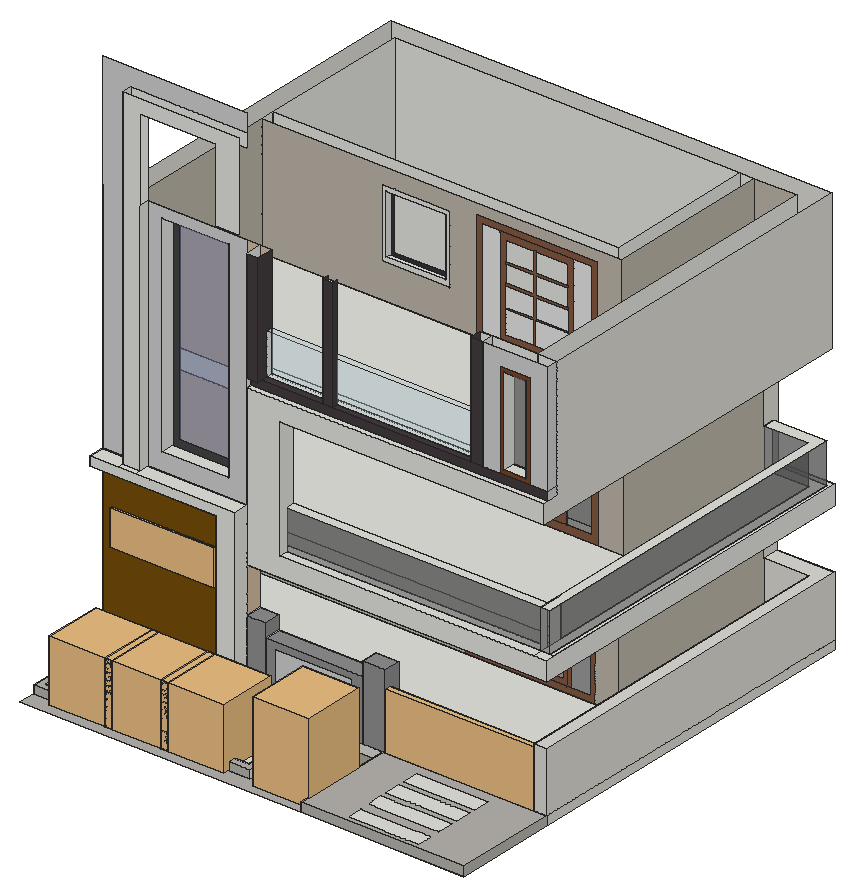
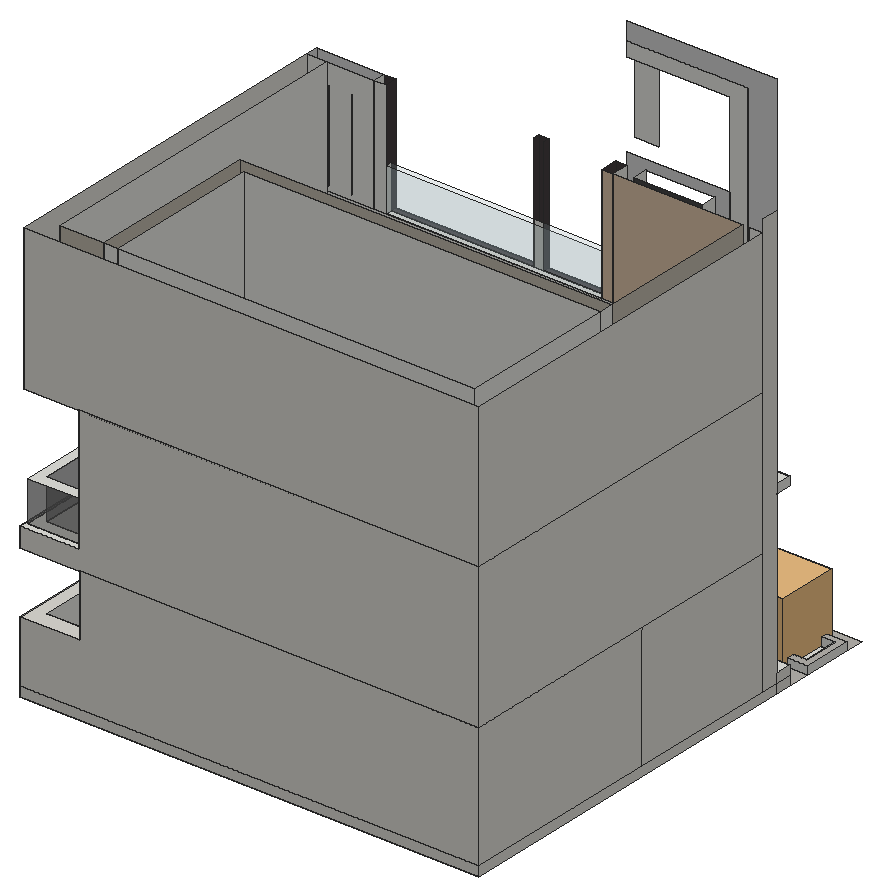
# SketchUp Ruby script. Lengths in inches.
U = 1.inch
M = Sketchup.active_model
def pt(a) = Geom::Point3d.new(a.map { |v| v * U })
def face(e, loops, mat)
  f = e.add_face(loops[0].map { |a| pt(a) })
  loops[1..].each { |l| e.add_face(l.map { |a| pt(a) }).erase! }
  f.material = f.back_material = mat if mat
  f
end
# faces: each face lists its corners as indices into pts; further lists are holes
def faces(e, pts, list, mat = nil) = list.each { |f| face(e, (f[0].is_a?(Array) ? f : [f]).map { |l| l.map { |i| pts[i] } }, mat) }
# xy, xz, yz: faces in a plane at the given z, y or x. An outline is a flat list of corners, or four numbers for a rectangle; further outlines are holes
def ring(l) = l.size == 4 ? [[l[0], l[1]], [l[2], l[1]], [l[2], l[3]], [l[0], l[3]]] : l.each_slice(2).to_a
def flat(e, list, mat, &to3) = list.each { |f| face(e, (f[0].is_a?(Array) ? f : [f]).map { |l| ring(l).map { |u, v| to3.(u, v) } }, mat) }
def xy(e, z, list, mat = nil) = flat(e, list, mat) { |x, y| [x, y, z] }
def xz(e, y, list, mat = nil) = flat(e, list, mat) { |x, z| [x, y, z] }
def yz(e, x, list, mat = nil) = flat(e, list, mat) { |y, z| [x, y, z] }
def lines(e, pts, list) = list.each { |a, b| e.add_line(pt(pts[a]), pt(pts[b])) }
# prism: a flat outline (further loops are holes) pulled along v
def prism(e, loops, v, mat = nil)
  f = face(e, loops, mat); d = Geom::Vector3d.new(v.map { |x| x * U })
  f.pushpull(f.normal.samedirection?(d) ? d.length : -d.length)
end
def box(e, o, s, mat = nil) = prism(e, [[o, [o[0] + s[0], o[1], o[2]], [o[0] + s[0], o[1] + s[1], o[2]], [o[0], o[1] + s[1], o[2]]]], [0, 0, s[2]], mat)
def at(x, y, z, deg = 0) = Geom::Transformation.translation(pt([x, y, z])) * Geom::Transformation.rotation(ORIGIN, Z_AXIS, deg.degrees)
def axes(o, x, y, z) = Geom::Transformation.new([*x, 0, *y, 0, *z, 0, *pt(o).to_a, 1])
def part(name) = M.definitions.add(name)
# library, detail: a bought-in or finely detailed component or shape, given as its bounding box
def library(name, o, s) = part(name).tap { |d| box(d.entities, o, s) }
def detail(e, o, s) = box(e.add_group.entities, o, s)
def put(e, d, t, mat = nil) = e.add_instance(d, t).tap { |i| i.material = mat if mat }
def group(e, t, mat = nil) = e.add_group.tap { |g| g.transformation = t; g.material = mat if mat }.entities
root = M.entities
M.materials.add("[Asphalt New]").color = [67, 60, 62]
M.materials.add("[Blinds Wood Light]").color = [119, 77, 10]
M.materials.add("[Carrera Marble]").color = [207, 207, 207]
M.materials.add("[Cinder Block]").color = [188, 181, 168]
M.materials.add("[Cladding Siding White]").color = [207, 207, 207]
M.materials.add("[Color M04]").color = [142, 142, 142]
M.materials.add("[Formica Beige]").color = [211, 187, 149]
M.materials.add("[Formica Graystone]").color = [149, 146, 135]
M.materials.add("[Formica Laminate Dark]").color = [50, 53, 60]
M.materials.add("[Formica Laminate Light]").color = [213, 189, 164]
M.materials.add("[Granite Dark Gray]").color = [69, 68, 68]
M.materials.add("[Mirror 01]").color = [155, 155, 155]
M.materials.add("[Mirror 02]").color = [229, 229, 229]
M.materials.add("[Terrazzo Tile Light]").color = [219, 217, 210]
M.materials.add("[Tile Travertine 2 inch]").color = [181, 178, 172]
M.materials.add("[Translucent Glass Block Dark]").color = [124, 124, 121]
M.materials["[Translucent Glass Block Dark]"].alpha = 0.8
M.materials.add("[Translucent Glass Gray]").color = [96, 96, 96]
M.materials["[Translucent Glass Gray]"].alpha = 0.5
M.materials.add("[Translucent Glass Gray]1").color = [56, 56, 56]
M.materials["[Translucent Glass Gray]1"].alpha = 0.5
M.materials.add("[Translucent Glass Safety]").color = [213, 245, 255]
M.materials["[Translucent Glass Safety]"].alpha = 0.21
M.materials.add("[Translucent Glass Sky Reflection]").color = [126, 138, 183]
M.materials["[Translucent Glass Sky Reflection]"].alpha = 0.52
M.materials.add("[Wood Veneer 01]").color = [120, 70, 37]
M.materials.add("[Wood Veneer 02]").color = [132, 89, 63]
c1 = library("chau cay",[-24.34,-109.24,0],[56.46,62.58,79.69])
c2 = library("Small+Bush+Planter",[-31.86,3.96,0],[62.63,58.8,106.375])
c3 = library("Gate_Lasercut_10ftx6ft_Kalil",[-0.15,-3.25,-0.15],[120,5.625,60.3])
c4 = library("WELCOMES YOU    ",[28.02,0,0],[211.02,85.69,12])
xy(root,0,[[280.73,0,444,102.9],[[0,17.14,216.1875,64.76],[6.6875,23.82,209.5,58.07]],[6.6875,23.82,209.5,58.07],[0,87.22,126.375,102.9],[126.375,87.22,144.47,102.9],
  [0,102.9,444,462.9]])
xy(root,0,[[144.47,87.22,280.73,102.9]],"[Formica Graystone]")
xy(root,0,[[0,0,0,17.14,216.1875,17.14,216.1875,64.76,0,64.76,0,87.22,280.73,87.22,280.73,0]],"[Tile Travertine 2 inch]")
xy(root,7.9375,[[[0,17.14,216.1875,64.76],[6.6875,23.82,209.5,58.07]]],"[Tile Travertine 2 inch]")
xy(root,9,[[323.27,4.95,394.4,21.2],[323.27,30.45,394.4,46.7],[323.27,52.89,394.4,69.14],[323.27,75.83,394.4,92.08],[431.59,102.9,431.59,446.14,12.41,446.14,12.41,265.43,0,265.43,0,462.9,444,462.9,444,102.9],
  [144.47,102.9,163.28,119.67],[163.28,102.9,260.1875,119.67],[260.1875,102.9,282.66,119.67],[282.66,102.9,431.59,119.67],[0,119.67,12.41,265.43],
  [12.41,119.67,431.59,119.67,431.59,446.14,386.49,446.14,386.49,265.43,12.41,265.43],[12.41,265.43,12.41,282.9,371.02,282.9,371.02,446.14,386.49,446.14,386.49,265.43],[12.41,282.9,371.02,446.14]])
xy(root,9,[[[280.73,0,444,102.9],[323.27,75.83,394.4,92.08],[323.27,52.89,394.4,69.14],[323.27,30.45,394.4,46.7],[323.27,4.95,394.4,21.2]]],"[Tile Travertine 2 inch]")
xy(root,18.75,[[0,87.22,126.375,102.9]])
xy(root,36.61,[[153.33,261.56,208.83,265.43]])
xy(root,41.66,[[157.07,261.56,205.1,265.43],[157.07,265.43,205.1,272.24]])
xy(root,69.0625,[[431.59,102.9,444,102.9,444,462.9,386.49,462.9,386.49,446.14,431.59,446.14]],"[Terrazzo Tile Light]")
xy(root,69.375,[[163.28,102.9,260.1875,119.67]],"[Color M04]")
xy(root,83.3125,[[144.47,102.9,163.28,119.67],[260.1875,102.9,282.66,119.67]],"[Color M04]")
xy(root,106.57,[[157.07,261.56,205.1,265.43],[157.07,265.43,205.1,272.24]])
xy(root,111.61,[[153.33,261.56,208.83,265.43]])
xy(root,129,[[0,265.43,12.41,282.9],[12.41,265.43,386.49,282.9],[0,282.9,12.41,446.14],[12.41,282.9,371.02,446.14],[371.02,282.9,386.49,446.14],
  [0,446.14,371.02,462.9],[371.02,446.14,386.49,462.9]])
xy(root,129,[[144.47,102.9,144.47,119.67,12.41,119.67,12.41,265.43,444,265.43,444,102.9],[386.49,265.43,444,282.9],[386.49,282.9,444,462.9]],"[Formica Laminate Light]")
xy(root,148.25,[[177.22,102.9,431.49,111.29],[431.49,102.9,444,111.29],[144.47,111.29,431.49,119.67],[431.49,111.29,431.49,446,387.1,446,387.1,457.35,440.93,457.35,440.93,111.29],[440.93,111.29,444,111.29,444,462.9,387.1,462.9,387.1,457.35,440.93,457.35],
  [12.51,119.67,431.49,136.57],[12.51,136.57,431.49,136.57,431.49,446,387.1,446,387.1,270.94,12.51,270.94],[12.51,270.94,12.51,291.29,374.49,291.29,374.49,446,387.1,446,387.1,270.94],[12.51,291.29,374.49,446]])
xy(root,173.4,[[0,87.22,126.375,102.9]])
xy(root,181.66,[[140.6875,266.5,207.375,270.94]])
xy(root,182.21,[[0,87.22,27.95,102.9],[27.95,87.22,45.1,93.15],[45.1,87.22,144.47,102.9],[27.95,93.15,45.1,102.9]])
xy(root,187.05,[[146.07,266.5,201.99,270.94],[146.07,270.94,201.99,276.82]])
xy(root,187.8125,[[144.47,111.29,177.22,119.67],[177.22,111.29,431.49,119.67],[431.49,111.29,440.93,111.29,440.93,457.35,387.1,457.35,387.1,446,431.49,446]])
xy(root,199.72,[[59.64,102.9,126.33,116.97]])
xy(root,242.97,[[146.07,266.5,201.99,270.94],[146.07,270.94,201.99,276.82]])
xy(root,248.35,[[140.6875,266.5,207.375,270.94]])
xy(root,268.25,[[0,119.67,12.51,136.57],[0,136.57,12.51,270.94],[0,270.94,12.51,291.29],[12.51,270.94,387.1,291.29],[0,291.29,12.51,446],
  [12.51,291.29,374.49,446],[374.49,291.29,387.1,446],[0,446,374.49,462.9],[374.49,446,387.1,462.9]])
xy(root,268.25,[[177.22,102.9,177.22,119.67,12.51,119.67,12.51,270.94,440.93,270.94,440.93,102.9],[387.1,270.94,440.93,291.29],[387.1,291.29,440.93,462.9]],"[Formica Laminate Light]")
xy(root,287.4375,[[144.47,102.9,440.93,107.86],[144.47,107.86,440.93,119.67],[19.52,119.67,421.41,139.1875],[19.52,139.1875,421.41,139.1875,421.41,443.38,378.85,443.38,378.85,278.02,19.52,278.02],[19.52,278.02,19.52,291.29,365.25,291.29,365.25,443.38,378.85,443.38,378.85,278.02],
  [19.52,291.29,365.25,443.38]])
xy(root,295.875,[[144.47,102.9,155.47,107.86],[144.47,107.86,155.47,119.67],[216.29,107.86,226.02,113.77],[364.18,107.86,376,119.67],[376,107.86,440.93,119.67],
  [155.47,113.77,364.18,119.67]])
xy(root,295.875,[[155.47,107.86,216.29,113.77],[226.02,107.86,364.18,113.77]],"[Asphalt New]")
xy(root,300.34,[[397.72,107.86,419.72,119.36]])
xy(root,327.01,[[143.73,278.02,202.85,283.21]])
xz(root,0,[[280.73,0,444,9]],"[Tile Travertine 2 inch]")
xz(root,17.14,[[0,0,216.1875,7.9375]],"[Tile Travertine 2 inch]")
xz(root,23.82,[[6.6875,0,209.5,7.9375]])
xz(root,58.07,[[6.6875,0,209.5,7.9375]],"[Tile Travertine 2 inch]")
xz(root,64.76,[[0,0,216.1875,7.9375]])
xz(root,87.22,[[0,0,126.375,18.75],[126.375,0,144.47,0,144.47,182.21,0,182.21,0,173.4,126.375,173.4]])
xz(root,93.15,[[27.95,182.21,45.1,182.21,45.1,501.96,121.39,501.96,121.39,428.03,144.47,428.03,144.47,515.65,27.95,515.65]])
xz(root,102.9,[[0,0,126.375,18.75],[126.375,0,126.375,173.4,0,173.4,0,182.21,144.47,182.21,144.47,0],[280.73,0,444,9],[144.47,129,444,129,444,148.25,177.22,148.25,177.22,268.25,440.93,268.25,440.93,287.4375,144.47,287.4375],[27.95,182.21,27.95,515.65,144.47,515.65,144.47,501.96,45.1,501.96,45.1,182.21]])
xz(root,102.9,[[144.47,295.875,155.47,407.4375]],"[Asphalt New]")
xz(root,102.9,[[0,18.75,126.375,173.4]],"[Blinds Wood Light]")
xz(root,102.9,[[172.84,16.04,248.99,63.1]],"[Carrera Marble]")
xz(root,102.9,[[0,182.21,27.95,182.21,27.95,515.65,144.47,515.65,144.47,533.5625,0,533.5625],[[45.1,182.21,144.47,419.375],[59.64,199.72,126.33,409.91]]],"[Cladding Siding White]")
xz(root,102.9,[[144.47,9,163.28,83.3125],[[163.28,9,260.1875,69.375],[172.84,16.04,248.99,63.1]],[260.1875,9,282.66,83.3125]],"[Color M04]")
xz(root,102.9,[[144.47,0,280.73,9],[431.59,9,444,69.0625]],"[Terrazzo Tile Light]")
xz(root,107.86,[[144.47,287.4375,440.93,295.875],[216.29,295.875,226.02,407.4375],[364.18,295.875,376,407.4375]],"[Asphalt New]")
xz(root,107.86,[[376,295.875,393.25,295.875,393.25,392.4375,424.1875,392.4375,424.1875,295.875,440.93,295.875,440.93,407.4375,376,407.4375]],"[Carrera Marble]")
xz(root,107.86,[[[393.25,295.875,424.1875,392.4375],[397.72,300.34,419.72,387.97]]],"[Wood Veneer 01]")
xz(root,111.29,[[144.47,148.25,177.22,187.8125]])
xz(root,111.29,[[177.22,148.25,431.49,187.8125],[431.49,148.25,440.93,187.8125]],"[Translucent Glass Gray]")
xz(root,113.77,[[216.29,295.875,226.02,337.375]])
xz(root,113.77,[[155.47,295.875,216.29,337.375],[226.02,295.875,364.18,337.375]],"[Translucent Glass Safety]")
xz(root,116.97,[[[59.64,199.72,126.33,409.91],[66.47,206.55,119.51,403.08]]],"[Granite Dark Gray]")
xz(root,116.97,[[66.47,206.55,119.51,403.08]],"[Translucent Glass Sky Reflection]")
xz(root,119.36,[[397.72,300.34,419.72,387.97]],"[Translucent Glass Block Dark]")
xz(root,119.67,[[0,9,12.41,129],[260.1875,9,282.66,83.3125],[0,129,12.41,268.25],[12.41,129,144.47,129,144.47,148.25,12.51,148.25,12.51,268.25,12.41,268.25],[0,268.25,12.41,287.4375],
  [12.41,268.25,12.51,287.4375],[12.51,268.25,144.47,287.4375],[0,287.4375,12.41,407.4375],[12.41,287.4375,12.51,407.4375],[144.47,287.4375,421.41,295.875],
  [421.41,287.4375,440.93,295.875],[364.18,295.875,376,407.4375],[376,295.875,421.41,407.4375],[421.41,295.875,440.93,407.4375]])
xz(root,119.67,[[144.47,9,163.28,83.3125],[163.28,9,260.1875,69.375]],"[Color M04]")
xz(root,119.67,[[12.41,9,144.47,129],[12.51,148.25,144.47,268.25],[144.47,187.8125,177.22,268.25],[19.52,287.4375,144.47,407.4375],[144.47,295.875,155.47,407.4375]],"[Formica Laminate Light]")
xz(root,119.67,[[144.47,148.25,431.49,187.8125]],"[Translucent Glass Gray]")
xz(root,119.67,[[155.47,295.875,364.18,337.375]],"[Translucent Glass Safety]")
xz(root,261.56,[[[153.33,36.61,208.83,111.61],[157.07,41.66,205.1,106.57]]])
xz(root,265.43,[[0,9,12.41,129],[[153.33,36.61,208.83,111.61],[157.07,41.66,205.1,106.57]]])
xz(root,265.43,[[[12.41,9,232.01,9,232.01,117.875,362.37,117.875,362.37,9,386.49,9,386.49,129,12.41,129],[153.33,36.61,208.83,111.61]]],"[Cinder Block]")
xz(root,265.43,[[236.38,14.91,256.62,86.9],[338.81,14.91,357.99,86.9],[264.98,21.42,294.21,45.24],[297.63,21.42,329.84,45.24],[264.98,47.89,294.21,66.625],
  [297.63,47.89,329.84,66.625],[264.98,69.28,294.21,83.67],[297.63,69.28,329.84,83.67],[264.98,86.3125,294.21,105.46],[297.63,86.3125,329.84,105.46],
  [236.38,90.91,256.62,111.96],[338.81,90.91,357.99,111.96]],"[Mirror 01]")
xz(root,265.43,[[[232.01,9,362.37,117.875],[236.38,14.91,357.99,111.96]],[256.62,14.91,260.17,111.96],[[260.17,14.91,334.65,111.96],[264.98,21.42,329.84,105.46]],[334.65,14.91,338.81,111.96],[294.21,21.42,297.63,21.42,297.63,45.24,329.84,45.24,329.84,47.89,297.63,47.89,297.63,66.625,329.84,66.625,329.84,69.28,297.63,69.28,297.63,83.67,329.84,83.67,329.84,86.3125,297.63,86.3125,297.63,105.46,294.21,105.46,294.21,86.3125,264.98,86.3125,264.98,83.67,294.21,83.67,294.21,69.28,264.98,69.28,264.98,66.625,294.21,66.625,294.21,47.89,264.98,47.89,264.98,45.24,294.21,45.24],
  [236.38,86.9,256.62,90.91],[338.81,86.9,357.99,90.91]],"[Wood Veneer 02]")
xz(root,266.5,[[[140.6875,181.66,207.375,248.35],[146.07,187.05,201.99,242.97]]])
xz(root,270.94,[[[140.6875,181.66,207.375,248.35],[146.07,187.05,201.99,242.97]]])
xz(root,270.94,[[[12.51,148.25,232.73,148.25,232.73,260.24,361.8125,260.24,361.8125,148.25,387.1,148.25,387.1,268.25,12.51,268.25],[140.6875,181.66,207.375,248.35]]],"[Cinder Block]")
xz(root,270.94,[[240.11,155.63,264.98,252.85],[329.84,155.63,354.43,252.85],[271.55,162.2,294.96,183.96],[297.16,162.2,323.27,183.96],[271.55,185.89,294.96,204.33],
  [297.16,185.89,323.27,204.33],[271.55,206.15,294.96,223.48],[297.16,206.15,323.27,223.48],[271.55,224.83,294.96,246.29],[297.16,224.83,323.27,246.29]],"[Translucent Glass Gray]1")
xz(root,270.94,[[[232.73,148.25,361.8125,260.24],[240.11,155.63,354.43,252.85]],[[264.98,155.63,329.84,252.85],[271.55,162.2,323.27,246.29]],[294.96,162.2,297.16,162.2,297.16,183.96,323.27,183.96,323.27,185.89,297.16,185.89,297.16,204.33,323.27,204.33,323.27,206.15,297.16,206.15,297.16,223.48,323.27,223.48,323.27,224.83,297.16,224.83,297.16,246.29,294.96,246.29,294.96,224.83,271.55,224.83,271.55,223.48,294.96,223.48,294.96,206.15,271.55,206.15,271.55,204.33,294.96,204.33,294.96,185.89,271.55,185.89,271.55,183.96,294.96,183.96]],"[Wood Veneer 02]")
xz(root,272.24,[[[157.07,41.66,205.1,106.57],[159.51,44.96,202.65,103.26]],[178.86,44.96,181.3,103.26]],"[Formica Laminate Dark]")
xz(root,272.24,[[159.51,44.96,178.86,103.26],[181.3,44.96,202.65,103.26]],"[Translucent Glass Gray]")
xz(root,276.82,[[[146.07,187.05,201.99,242.97],[149.23,190.21,198.83,239.8]],[172.41,190.21,175,239.8]],"[Formica Laminate Dark]")
xz(root,276.82,[[149.23,190.21,172.41,239.8],[175,190.21,198.83,239.8]],"[Translucent Glass Gray]")
xz(root,278.02,[[[138.88,322.17,207.69,390.98],[143.73,327.01,202.85,386.13]]])
xz(root,278.02,[[[19.52,287.4375,232.96,287.4375,232.96,397.1875,355.14,397.1875,355.14,287.4375,378.85,287.4375,378.85,407.4375,19.52,407.4375],[138.88,322.17,207.69,390.98]]],"[Cinder Block]")
xz(root,278.02,[[238.99,293.47,257.2,391.15],[331.25,293.47,349.11,391.15],[263.57,299.85,290.95,322.42],[292.74,299.85,324.88,322.42],[263.57,323.98,290.95,343.25],
  [292.74,323.98,324.88,343.25]],"[Mirror 02]")
xz(root,278.02,[[[232.96,287.4375,355.14,397.1875],[238.99,293.47,349.11,391.15]],[[257.2,293.47,331.25,391.15],[263.57,299.85,324.88,384.78]],[290.95,299.85,292.74,299.85,292.74,322.42,324.88,322.42,324.88,323.98,292.74,323.98,292.74,343.25,324.88,343.25,324.88,345.67,292.74,345.67,292.74,362.74,324.88,362.74,324.88,365.24,292.74,365.24,292.74,384.78,290.95,384.78,290.95,365.24,263.57,365.24,263.57,362.74,290.95,362.74,290.95,345.67,263.57,345.67,263.57,343.25,290.95,343.25,290.95,323.98,263.57,323.98,263.57,322.42,290.95,322.42]],"[Wood Veneer 02]")
xz(root,282.9,[[12.41,9,371.02,129]])
xz(root,283.21,[[[143.73,327.01,202.85,386.13],[146.7,329.99,199.875,383.16]]],"[Formica Laminate Dark]")
xz(root,291.29,[[12.51,148.25,374.49,268.25],[19.52,287.4375,365.25,407.4375]])
xz(root,443.38,[[19.52,287.4375,365.25,407.4375],[365.25,287.4375,378.85,407.4375]])
xz(root,443.38,[[378.85,287.4375,421.41,407.4375]],"[Cinder Block]")
xz(root,446,[[12.51,148.25,374.49,268.25],[374.49,148.25,387.1,268.25]])
xz(root,446,[[387.1,148.25,431.49,187.8125]],"[Translucent Glass Gray]")
xz(root,446.14,[[12.41,9,371.02,129],[371.02,9,386.49,129]])
xz(root,446.14,[[386.49,9,431.59,69.0625]],"[Terrazzo Tile Light]")
xz(root,457.35,[[387.1,148.25,440.93,187.8125]],"[Translucent Glass Gray]")
xz(root,462.9,[[0,0,444,9],[0,9,0,129,386.49,129,386.49,69.0625,444,69.0625,444,9],[0,129,0,268.25,387.1,268.25,387.1,148.25,444,148.25,444,129],[0,268.25,440.93,407.4375]],"[Terrazzo Tile Light]")
yz(root,0,[[17.14,0,64.76,7.9375],[87.22,173.4,102.9,182.21]])
yz(root,0,[[87.22,0,102.9,9],[102.9,0,462.9,9],[87.22,9,102.9,18.75],[102.9,9,119.67,419.375],[119.67,9,265.43,129],
  [265.43,9,462.9,129],[119.67,129,462.9,268.25],[119.67,268.25,462.9,407.4375]],"[Terrazzo Tile Light]")
yz(root,6.6875,[[23.82,0,58.07,7.9375]])
yz(root,12.41,[[265.43,9,282.9,129],[282.9,9,446.14,129]])
yz(root,12.41,[[119.67,9,265.43,129]],"[Cinder Block]")
yz(root,12.51,[[270.94,148.25,291.29,268.25],[291.29,148.25,446,268.25]])
yz(root,12.51,[[136.57,148.25,270.94,268.25]],"[Cinder Block]")
yz(root,12.51,[[119.67,148.25,136.57,268.25]],"[Formica Laminate Light]")
yz(root,19.52,[[278.02,287.4375,291.29,407.4375],[291.29,287.4375,443.38,407.4375]])
yz(root,19.52,[[119.67,287.4375,278.02,407.4375]],"[Cinder Block]")
yz(root,27.95,[[93.15,182.21,102.9,515.65]])
yz(root,45.1,[[93.15,182.21,102.9,419.375]])
yz(root,59.64,[[102.9,199.72,116.97,409.91]])
yz(root,126.33,[[102.9,199.72,116.97,409.91]])
yz(root,126.375,[[87.22,0,102.9,9],[87.22,9,102.9,18.75],[87.22,18.75,102.9,173.4]])
yz(root,140.6875,[[266.5,181.66,270.94,248.35]])
yz(root,143.73,[[278.02,327.01,283.21,386.13]])
yz(root,144.47,[[87.22,0,102.9,9],[87.22,9,102.9,182.21],[102.9,9,119.67,83.3125],[102.9,129,119.67,148.25],[102.9,148.25,102.9,268.25,119.67,268.25,119.67,187.8125,111.29,187.8125,111.29,148.25],
  [111.29,148.25,119.67,187.8125],[102.9,268.25,119.67,287.4375],[102.9,287.4375,107.86,295.875],[107.86,287.4375,119.67,295.875],[102.9,295.875,119.67,407.4375]])
yz(root,144.47,[[102.9,83.3125,119.67,129]],"[Formica Laminate Light]")
yz(root,146.07,[[266.5,187.05,270.94,242.97],[270.94,187.05,276.82,242.97]])
yz(root,153.33,[[261.56,36.61,265.43,111.61]])
yz(root,155.47,[[113.77,295.875,119.67,337.375]])
yz(root,155.47,[[102.9,295.875,113.77,295.875,113.77,337.375,119.67,337.375,119.67,407.4375,102.9,407.4375]],"[Asphalt New]")
yz(root,157.07,[[261.56,41.66,265.43,106.57],[265.43,41.66,272.24,106.57]])
yz(root,163.28,[[102.9,9,119.67,69.375]])
yz(root,163.28,[[102.9,69.375,119.67,83.3125]],"[Color M04]")
yz(root,177.22,[[102.9,148.25,111.29,148.25,111.29,187.8125,119.67,187.8125,119.67,268.25,102.9,268.25]])
yz(root,201.99,[[266.5,187.05,270.94,242.97],[270.94,187.05,276.82,242.97]])
yz(root,202.85,[[278.02,327.01,283.21,386.13]])
yz(root,205.1,[[261.56,41.66,265.43,106.57],[265.43,41.66,272.24,106.57]])
yz(root,207.375,[[266.5,181.66,270.94,248.35]])
yz(root,208.83,[[261.56,36.61,265.43,111.61]])
yz(root,209.5,[[23.82,0,58.07,7.9375]])
yz(root,216.1875,[[17.14,0,64.76,7.9375]])
yz(root,216.29,[[107.86,295.875,113.77,407.4375]],"[Asphalt New]")
yz(root,226.02,[[107.86,295.875,113.77,407.4375]],"[Asphalt New]")
yz(root,260.1875,[[102.9,9,119.67,69.375],[102.9,69.375,119.67,83.3125]])
yz(root,280.73,[[87.22,0,102.9,9]])
yz(root,280.73,[[0,0,87.22,9]],"[Tile Travertine 2 inch]")
yz(root,282.66,[[102.9,9,119.67,83.3125]],"[Color M04]")
yz(root,364.18,[[113.77,295.875,119.67,337.375]])
yz(root,364.18,[[107.86,295.875,107.86,407.4375,119.67,407.4375,119.67,337.375,113.77,337.375,113.77,295.875]],"[Asphalt New]")
yz(root,365.25,[[291.29,287.4375,443.38,407.4375]])
yz(root,371.02,[[282.9,9,446.14,129]])
yz(root,374.49,[[291.29,148.25,446,268.25]])
yz(root,376,[[107.86,295.875,119.67,407.4375]])
yz(root,378.85,[[278.02,287.4375,443.38,407.4375]],"[Cinder Block]")
yz(root,386.49,[[265.43,9,446.14,129]],"[Cinder Block]")
yz(root,386.49,[[446.14,69.0625,462.9,129]],"[Terrazzo Tile Light]")
yz(root,387.1,[[446,148.25,457.35,187.8125]])
yz(root,387.1,[[270.94,148.25,446,268.25]],"[Cinder Block]")
yz(root,387.1,[[457.35,148.25,462.9,148.25,462.9,268.25,446,268.25,446,187.8125,457.35,187.8125]],"[Terrazzo Tile Light]")
yz(root,397.72,[[107.86,300.34,119.36,387.97]])
yz(root,419.72,[[107.86,300.34,119.36,387.97]])
yz(root,421.41,[[119.67,287.4375,443.38,407.4375]])
yz(root,431.49,[[111.29,148.25,119.67,187.8125],[119.67,148.25,136.57,187.8125]])
yz(root,431.49,[[136.57,148.25,446,187.8125]],"[Translucent Glass Gray]")
yz(root,431.59,[[102.9,9,119.67,69.0625],[119.67,9,446.14,69.0625]])
yz(root,440.93,[[107.86,287.4375,119.67,295.875],[107.86,295.875,119.67,407.4375]],"[Carrera Marble]")
yz(root,440.93,[[102.9,268.25,462.9,268.25,462.9,407.4375,119.67,407.4375,119.67,287.4375,102.9,287.4375]],"[Terrazzo Tile Light]")
yz(root,440.93,[[111.29,148.25,457.35,187.8125]],"[Translucent Glass Gray]")
yz(root,444,[[102.9,129,462.9,148.25]])
yz(root,444,[[102.9,0,462.9,9],[102.9,9,462.9,69.0625]],"[Terrazzo Tile Light]")
yz(root,444,[[0,0,102.9,9]],"[Tile Travertine 2 inch]")
put(root,c1,at(249.1875,118.78,0))
put(root,c2,axes([108.09,7.2,0],[1,0,0],[0,1,0],[0,0,0.576]))
put(root,c2,axes([163.78,7.2,0],[1,0,0],[0,1,0],[0,0,0.576]))
put(root,c2,axes([52.03,7.2,0],[1,0,0],[0,1,0],[0,0,0.576]))
put(root,c3,axes([282.84,106.09,9.14],[1.24079,0,0],[0,1,0],[0,0,0.94751]))
put(root,c4,axes([-3.9,102.9,98.55],[0.4895,0,0],[0,0,0.41],[0,-0.23,0]),"[Formica Beige]")
